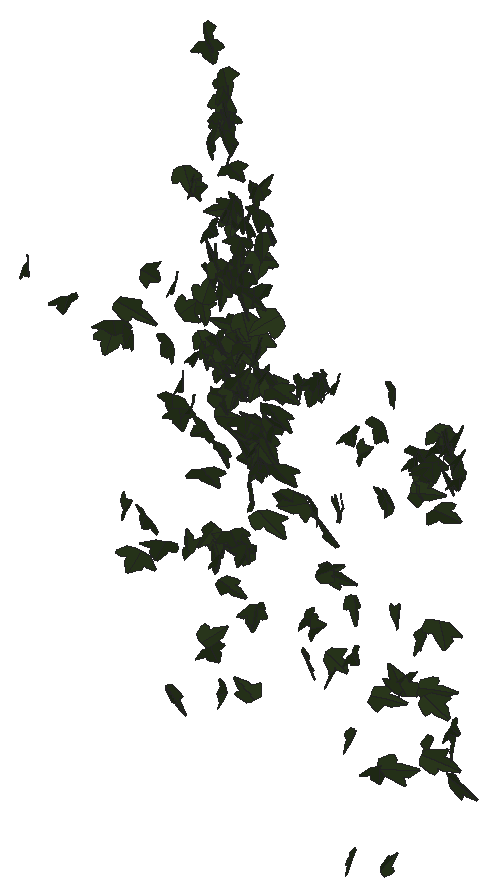
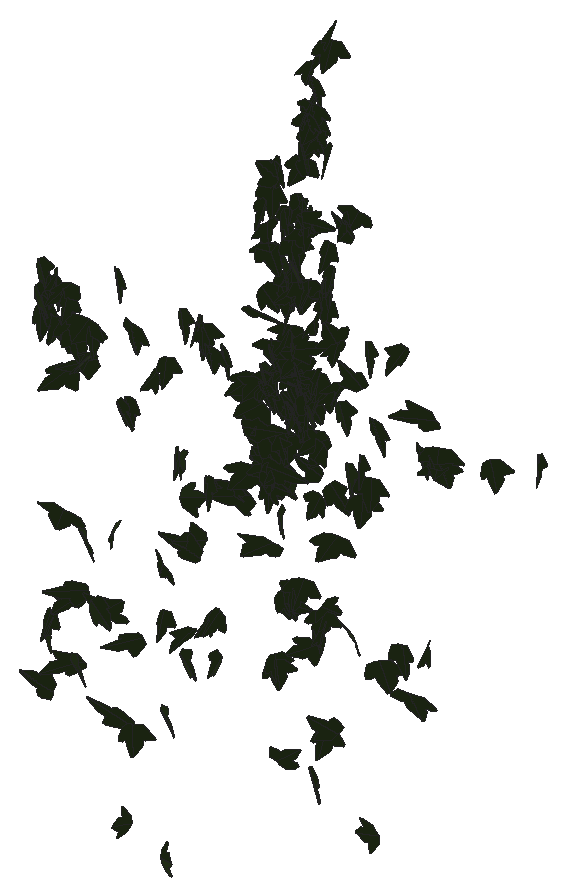
# SketchUp Ruby script. Lengths in millimetres.
U = 1.mm
M = Sketchup.active_model
def pt(a) = Geom::Point3d.new(a.map { |v| v * U })
def face(e, loops, mat)
  f = e.add_face(loops[0].map { |a| pt(a) })
  loops[1..].each { |l| e.add_face(l.map { |a| pt(a) }).erase! }
  f.material = f.back_material = mat if mat
  f
end
# faces: each face lists its corners as indices into pts; further lists are holes
def faces(e, pts, list, mat = nil) = list.each { |f| face(e, (f[0].is_a?(Array) ? f : [f]).map { |l| l.map { |i| pts[i] } }, mat) }
# xy, xz, yz: faces in a plane at the given z, y or x. An outline is a flat list of corners, or four numbers for a rectangle; further outlines are holes
def ring(l) = l.size == 4 ? [[l[0], l[1]], [l[2], l[1]], [l[2], l[3]], [l[0], l[3]]] : l.each_slice(2).to_a
def flat(e, list, mat, &to3) = list.each { |f| face(e, (f[0].is_a?(Array) ? f : [f]).map { |l| ring(l).map { |u, v| to3.(u, v) } }, mat) }
def xy(e, z, list, mat = nil) = flat(e, list, mat) { |x, y| [x, y, z] }
def xz(e, y, list, mat = nil) = flat(e, list, mat) { |x, z| [x, y, z] }
def yz(e, x, list, mat = nil) = flat(e, list, mat) { |y, z| [x, y, z] }
def lines(e, pts, list) = list.each { |a, b| e.add_line(pt(pts[a]), pt(pts[b])) }
# prism: a flat outline (further loops are holes) pulled along v
def prism(e, loops, v, mat = nil)
  f = face(e, loops, mat); d = Geom::Vector3d.new(v.map { |x| x * U })
  f.pushpull(f.normal.samedirection?(d) ? d.length : -d.length)
end
def box(e, o, s, mat = nil) = prism(e, [[o, [o[0] + s[0], o[1], o[2]], [o[0] + s[0], o[1] + s[1], o[2]], [o[0], o[1] + s[1], o[2]]]], [0, 0, s[2]], mat)
def at(x, y, z, deg = 0) = Geom::Transformation.translation(pt([x, y, z])) * Geom::Transformation.rotation(ORIGIN, Z_AXIS, deg.degrees)
def axes(o, x, y, z) = Geom::Transformation.new([*x, 0, *y, 0, *z, 0, *pt(o).to_a, 1])
def part(name) = M.definitions.add(name)
# library, detail: a bought-in or finely detailed component or shape, given as its bounding box
def library(name, o, s) = part(name).tap { |d| box(d.entities, o, s) }
def detail(e, o, s) = box(e.add_group.entities, o, s)
def put(e, d, t, mat = nil) = e.add_instance(d, t).tap { |i| i.material = mat if mat }
def group(e, t, mat = nil) = e.add_group.tap { |g| g.transformation = t; g.material = mat if mat }.entities
root = M.entities
M.materials.add("efeu2").color = [43, 57, 29]
c1 = part("ivyleaf_10")
p = [[0,12.8,-0.8],[-1.5,51.3,-10.9],[-4.9,51,-11.6],[-13.6,26.5,-7.3],[-13.2,15.9,-4.6],[-21.1,19.3,-7.2],
  [-29.5,16.3,-8.3],[-29.2,8.3,-6.2],[-19.7,-9.8,0.5],[-7.6,-13,4],[1,-12.2,5.8],[-0.4,51.1,-11.1],
  [-1.5,51.1,-10.9],[1,-12.4,5.9],[16.9,-12.4,3.5],[35.1,9.1,-5.1],[35,12.9,-6.1],[20.5,16.4,-4.9],
  [15.8,15,-3.8],[15.3,27.6,-7.1],[12.8,31.3,-7.8]]
faces(c1.entities,p,[[0,1,2,3,4,5,6,7,8,9,10],[11,12,0,13,14,15,16,17,18,19,20]],"efeu2")
put(root,c1,axes([392.9,1061.3,793.9],[0.22328,-0.58138,-0.2462],[0.15253,0.26211,-0.58075],[1.1919,0.07537,0.12044]))
put(root,c1,axes([469.6,1064.6,759.5],[-0.40368,-0.59835,-0.04185],[0.01906,0.04086,-0.63482],[1.1414,-0.2123,-0.0042]))
put(root,c1,axes([556.4,1064.1,726.9],[0.80132,0.45198,-0.16049],[-0.25562,-0.09391,-0.61682],[-0.87632,0.44069,0.03316]))
put(root,c1,axes([561.7,1063.9,746.8],[-0.80907,-0.46934,-0.09728],[0.14828,0.06064,-0.63302],[0.90009,-0.43186,0.01684]))
put(root,c1,axes([585,1057,439.4],[0.06877,-0.15139,-0.63183],[0.06726,0.63232,-0.14948],[1.2347,-0.02602,0.04333]))
put(root,c1,axes([589.1,1063.6,739.4],[0.76379,-0.46532,-0.1728],[-0.03848,0.2067,-0.60357],[0.9439,0.38495,0.11522]))
put(root,c1,axes([607.7,1062.6,361.6],[1.193,-0.04431,-0.10252],[-0.19466,0.00702,-0.6284],[0.08538,0.63513,-0.0002]))
put(root,c1,axes([585.9,1058.6,789.2],[0.43486,0.10897,0.60259],[1.0456,0.24761,-0.25309],[-0.51477,0.59499,-0.00503]))
put(root,c1,axes([622.1,1067,428.7],[-0.86457,0.31996,0.33371],[-0.55477,0.16492,-0.55492],[-0.68296,-0.53901,0.02831]))
put(root,c1,axes([635.3,1050.3,868.7],[0.12233,0.43176,0.51307],[-0.17473,0.51623,-0.42292],[-1.2642,-0.02957,0.1081]))
put(root,c1,axes([654,1068.2,393.3],[-0.77826,-0.47441,0.11149],[-0.12473,-0.09068,-0.62625],[0.91906,-0.41403,0.00942]))
put(root,c1,axes([668.9,1061.3,749.4],[0.7785,-0.43948,-0.31281],[-0.20694,0.31734,-0.58803],[1.00559,0.40554,0.12116]))
put(root,c1,axes([678.7,1062.8,658.7],[-0.84104,-0.1225,0.08321],[-0.09056,-0.05701,-0.69887],[0.15634,-0.69204,0.04284]))
put(root,c1,axes([680.3,1062.5,864.1],[0.16723,-0.62621,-0.30183],[-0.09446,0.29198,-0.64093],[0.84282,0.15698,-0.01195]))
put(root,c1,axes([665.8,1073.2,138.9],[-0.44881,0.29664,-0.51951],[0.58109,-0.42054,-0.37872],[-0.97912,-0.38556,0.01337]))
put(root,c1,axes([685.9,1069.2,634.1],[-0.59843,-0.48389,-0.056],[0.06209,0.02813,-0.68884],[0.59103,-0.4929,0.01566]))
put(root,c1,axes([688.2,1068.5,691.8],[0.1738,-0.5851,-0.3012],[0.09152,0.30921,-0.58608],[1.24911,0.05876,0.08485]))
put(root,c1,axes([691.2,1072.2,811.6],[0.62877,-0.01901,-0.45169],[0.54909,-0.04296,0.51536],[-0.05196,-0.68396,-0.01982]))
put(root,c1,axes([715.1,1054.2,410.7],[0.54478,-0.018,0.5821],[-0.58554,0.40411,0.38067],[-0.40244,-0.61232,0.23412]))
put(root,c1,axes([698.8,1062.4,1059.8],[0.72653,0.1688,0.28357],[0.32911,0.08796,-0.61889],[-0.23189,0.65369,0.01006]))
put(root,c1,axes([711.3,1076.8,1048.2],[-0.05253,0.44145,-0.49501],[-0.08526,-0.49631,-0.43653],[-0.80468,0.02377,0.07857]))
put(root,c1,axes([716.4,1058.1,665.1],[0.0959,-0.56776,-0.30934],[-0.05063,0.30819,-0.57],[1.2295,0.05698,0.00066]))
put(root,c1,axes([705.4,1074.6,1034.9],[0.26849,-0.13751,-0.61151],[0.61981,-0.34043,0.25939],[-0.44783,-0.55361,-0.00761]))
put(root,c1,axes([726.4,1061.4,756.1],[-0.03635,-0.63454,-0.11075],[-0.02695,0.11119,-0.63459],[1.22561,-0.01637,-0.01724]))
put(root,c1,axes([741.9,1060.7,627.3],[-0.50209,-0.0235,0.53432],[-0.65103,-0.02726,-0.41222],[0.04385,-0.67389,-0.00195]))
put(root,c1,axes([734.3,1058.4,787.1],[0.20787,0.6266,0.06189],[-0.00518,0.06328,-0.6359],[-1.19833,0.10842,0.01348]))
put(root,c1,axes([736.9,1059.4,845.7],[0.12372,0.63143,0.01278],[-0.002,0.01321,-0.63951],[-0.7705,0.10135,0.00371]))
put(root,c1,axes([747,1063.4,940.4],[-0.5422,0.30795,0.35546],[-0.34994,0.21008,-0.54064],[-0.4547,-0.5289,-0.00778]))
put(root,c1,axes([737.9,1061.6,857.1],[0.39649,0.52898,-0.35342],[0.23779,0.29499,0.62075],[0.73881,-0.37882,-0.01013]))
put(root,c1,axes([738.6,1063,552.5],[-0.88042,-0.35241,-0.27711],[0.41422,0.17158,-0.58153],[0.74594,-0.51122,-0.00415]))
put(root,c1,axes([745.4,1060.9,954.8],[-0.57024,0.42153,0.17021],[-0.14614,0.1213,-0.62934],[-0.53501,-0.48242,-0.00952]))
put(root,c1,axes([742.6,1059.3,771.6],[0.11317,0.63243,-0.06084],[-0.09823,-0.0561,-0.63356],[-1.20521,0.06396,0.04593]))
put(root,c1,axes([743.5,1061.7,1324.2],[-0.24073,0.68446,0.04343],[-0.01136,0.04251,-0.71233],[-0.83664,-0.19752,-0.00282]))
put(root,c1,axes([745.2,1062.9,1297.6],[-0.5946,-0.48443,-0.14762],[0.16886,0.06966,-0.68556],[0.59431,-0.50445,0.04709]))
put(root,c1,axes([749.9,1063.5,905.3],[-0.73336,0.18282,0.11682],[-0.1341,0.04004,-0.62827],[-0.22819,-0.61105,-0.00621]))
put(root,c1,axes([748.7,1069.7,451.7],[0.23452,0.36446,-0.49963],[-0.26019,-0.45204,-0.41181],[-0.7082,0.28677,-0.01415]))
put(root,c1,axes([754.9,1054.3,1131.8],[-0.25245,0.39976,0.54185],[-0.37287,0.44934,-0.44822],[-0.73199,-0.36676,0.04145]))
put(root,c1,axes([750.5,1071.2,437.9],[-0.61943,-0.42061,-0.14316],[0.26525,-0.04563,-0.63706],[0.47272,-0.52555,0.16988]))
put(root,c1,axes([751.1,1072.8,416.5],[-0.10583,0.61072,-0.17549],[0.03365,-0.17333,-0.61684],[-0.77449,-0.09098,-0.00282]))
put(root,c1,axes([755,1054.4,985.6],[-0.08017,-0.50292,-0.45112],[0.07236,0.4472,-0.50719],[0.82105,-0.08852,0.00065]))
put(root,c1,axes([753.7,1078.6,1160],[0.16363,0.55805,-0.35439],[-0.13116,-0.33838,-0.57353],[-0.79576,0.17053,0.02166]))
put(root,c1,axes([762,1061,921.1],[-0.15887,0.29519,-0.60342],[-0.26362,0.56358,0.32233],[0.77598,0.25189,-0.01404]))
put(root,c1,axes([743.1,1061.5,263.6],[0.4158,0.20985,-0.55696],[0.59238,0.27314,0.40004],[0.41993,-0.59309,-0.01284]))
put(root,c1,axes([755.7,1057.9,251.7],[-0.43025,-0.55517,-0.29055],[0.25785,0.25826,-0.5989],[1.16435,-0.26234,0.02526]))
put(root,c1,axes([756,1072,689.7],[-0.71044,0.29558,-0.19809],[0.21399,-0.0921,-0.65304],[-0.3777,-0.60816,0.00262]))
put(root,c1,axes([764.5,1064.6,412.5],[0.08432,-0.65577,-0.06218],[-0.00676,0.06194,-0.6594],[0.8036,0.06933,0.00098]))
put(root,c1,axes([767.5,1062.7,789.6],[-0.80006,-0.02069,0.03525],[-0.04267,-0.00937,-0.65606],[0.02582,-0.65667,0.00825]))
put(root,c1,axes([767.8,1062.1,793.5],[-0.28795,0.50899,0.31432],[-0.19706,0.27113,-0.56034],[-0.70273,-0.28459,0.02834]))
put(root,c1,axes([761,1060.3,694.6],[0.29358,0.15755,0.56905],[0.2357,0.55966,-0.23664],[-0.6807,0.26174,0.16348]))
put(root,c1,axes([766.1,1064.2,605],[-0.69626,0.2669,-0.16946],[0.1823,-0.08047,-0.62996],[-0.33991,-0.58987,0.00926]))
put(root,c1,axes([781.1,1070.3,1023.7],[0.23337,0.08868,-0.65033],[-0.72864,-0.2574,-0.21077],[-0.33207,0.62711,0.00545]))
put(root,c1,axes([766.9,1071,877.1],[0.01214,0.56322,-0.30632],[0.00296,-0.30639,-0.56327],[-0.78218,0.00758,-0.00689]))
put(root,c1,axes([765.5,1071.8,1202.1],[0.83127,-0.00889,0.07959],[0.09713,0.00142,-0.68142],[0.01057,0.686,0.00244]))
put(root,c1,axes([777.8,1058.1,183.7],[0.28392,-0.45395,-0.49396],[-0.28257,0.47114,-0.47781],[1.24514,0.21043,0.0042]))
put(root,c1,axes([771.6,1065.3,747.6],[-0.58516,0.5382,0.14897],[-0.13809,0.13012,-0.61983],[-1.0538,-0.3159,-0.0015]))
put(root,c1,axes([772.6,1070.6,749.3],[-0.17042,0.33649,0.52486],[0.06826,-0.52893,0.354],[0.75755,0.12336,0.08617]))
put(root,c1,axes([773.1,1063.8,1235],[0.71357,-0.38305,-0.11515],[-0.0825,0.10636,-0.69728],[0.48096,0.58655,0.05124]))
put(root,c1,axes([779.7,1064.6,752.9],[-0.48282,-0.51057,0.28851],[-0.197,-0.23974,-0.64575],[0.68781,-0.42707,0.01757]))
put(root,c1,axes([771.7,1068.3,1178.9],[-0.7696,-0.25518,-0.17458],[0.22699,0.00349,-0.67742],[0.30125,-0.65452,0.06445]))
put(root,c1,axes([765.1,1077,732.3],[0.41577,-0.44059,-0.36727],[0.28085,-0.28622,0.55698],[-0.64095,-0.41122,0.00583]))
put(root,c1,axes([774,1069.1,1150.8],[-0.7642,0.27097,-0.10557],[0.08173,-0.10952,-0.67857],[-0.34524,-0.62572,0.07305]))
put(root,c1,axes([771.5,1074.5,1187.8],[0.72901,-0.29129,0.15191],[0.1723,-0.05691,-0.66468],[0.36187,0.61392,0.01046]))
put(root,c1,axes([761.3,1073,652.9],[0.25646,-0.04963,-0.60136],[0.70436,-0.1686,0.21573],[-0.21402,-0.61433,-0.01062]))
put(root,c1,axes([775,1067.2,1202],[-0.29686,0.63919,-0.06217],[0.01456,-0.06197,-0.68385],[-0.78336,-0.24338,0.01085]))
put(root,c1,axes([766.3,1058.7,921.1],[0.63936,0.15019,0.40597],[0.46734,0.13593,-0.54479],[-0.24591,0.64883,0.02016]))
put(root,c1,axes([777.7,1059.6,778.9],[-1.02579,-0.33163,-0.13671],[0.32068,-0.01623,-0.62491],[0.60267,-0.55581,0.09981]))
put(root,c1,axes([779.7,1073.5,1174.7],[-0.23363,0.5091,0.4197],[0.18122,-0.39254,0.54393],[0.78429,0.24236,-0.00065]))
put(root,c1,axes([777.1,1076.8,1109.3],[0.23756,-0.63629,-0.13979],[0.04709,-0.13438,0.66541],[-0.79339,-0.19849,-0.00237]))
put(root,c1,axes([795.1,1066.3,825.7],[-0.11304,-0.03208,-0.65813],[-0.75864,-0.21552,0.09806],[-0.26583,0.62871,0.00003]))
put(root,c1,axes([779.5,1060.3,1259],[0.07041,0.70095,0.01442],[0.00305,0.01426,-0.70332],[-0.85534,0.05775,-0.00132]))
put(root,c1,axes([786.9,1055.7,914.4],[-0.15792,0.28389,0.59825],[-0.32037,0.53759,-0.31192],[-0.74164,-0.29267,0.00736]))
put(root,c1,axes([783.8,1058.1,1013.7],[0.14046,-0.47739,0.43153],[-0.139,0.41633,0.49098],[-0.77269,-0.16167,-0.00988]))
put(root,c1,axes([787.9,1067.4,724.6],[-0.6433,0.41618,0.11689],[-0.16659,0.01458,-0.66787],[-0.50039,-0.5399,0.07207]))
put(root,c1,axes([783.2,1071.4,1007.4],[0.44064,0.5389,-0.07464],[-0.04636,-0.06438,-0.64873],[-0.66211,0.36315,-0.00424]))
put(root,c1,axes([801.9,1055.1,1018.1],[-0.08021,0.01768,0.64973],[-0.76433,0.1722,-0.06808],[-0.21119,-0.62994,-0.00037]))
put(root,c1,axes([793,1060.8,913.8],[-0.7415,-0.23896,0.03297],[-0.03543,-0.01623,-0.65306],[0.29215,-0.60847,0.00447]))
put(root,c1,axes([782.9,1061.9,776.9],[0.77544,0.46805,0.16624],[0.1815,0.1373,-0.6203],[-0.92772,0.41808,0.01759]))
put(root,c1,axes([781.5,1058.6,375.6],[-0.4603,-0.06423,-0.52016],[0.63382,0.03877,-0.38162],[0.0844,-0.64141,0.02902]))
put(root,c1,axes([790.4,1067.7,710.9],[0.82191,0.02357,-0.00614],[-0.00652,-0.02288,-0.67373],[-0.029,0.67334,-0.02268]))
put(root,c1,axes([794.1,1066.3,1037.3],[0.03141,0.53188,-0.34971],[-0.15073,-0.33917,-0.52493],[-0.76182,0.08904,0.08944]))
put(root,c1,axes([802.6,1059.4,1044.1],[-0.6156,0.26111,0.3322],[-0.42688,0.03184,-0.55651],[-0.28897,-0.60329,0.11441]))
put(root,c1,axes([793.2,1059.7,1103.2],[-0.54905,-0.36453,-0.3079],[0.28174,0.20398,-0.57904],[0.50942,-0.5057,-0.01161]))
put(root,c1,axes([795.4,1060.6,464.7],[-0.6033,-0.47064,-0.21459],[0.22205,0.11957,-0.68166],[0.59069,-0.52563,0.03708]))
put(root,c1,axes([800.5,1066,793.6],[0.40324,-0.5172,-0.22841],[-0.13116,0.20225,-0.61355],[0.67719,0.34715,0.01717]))
put(root,c1,axes([806.4,1064.8,971.8],[0.43366,-0.15738,-0.51242],[-0.3594,0.45631,-0.3445],[0.54635,0.42509,0.1801]))
put(root,c1,axes([790,1074.9,937.2],[-0.0351,-0.22617,-0.60564],[0.43311,-0.51218,0.17441],[-0.65917,-0.32449,0.14684]))
put(root,c1,axes([816.7,1069.4,436.1],[0.04863,0.04852,-0.64974],[-0.79459,0.02068,-0.03841],[0.02163,0.65063,0.04968]))
put(root,c1,axes([807.4,1063.2,977.8],[-0.58937,-0.39821,0.12112],[-0.11654,-0.07454,-0.62605],[0.49424,-0.49243,-0.00318]))
put(root,c1,axes([810.7,1055,821.9],[0.19771,-0.13127,0.63158],[-0.61394,0.54341,0.166],[-1.06318,-0.33821,0.02159]))
put(root,c1,axes([795.1,1057.1,804.7],[0.44567,0.40188,0.4552],[0.1708,0.45962,-0.45195],[-1.14298,0.22539,0.10996]))
put(root,c1,axes([802.3,1067.1,722.9],[0.53399,-0.51157,0.11609],[0.07989,-0.09673,-0.67314],[0.63497,0.44238,-0.01294]))
put(root,c1,axes([804.8,1073.3,711.3],[-0.45505,0.49609,0.18125],[0.1256,-0.14935,0.62062],[0.632,0.38687,0.00717]))
put(root,c1,axes([806.9,1064.1,782.1],[0.35691,-0.60033,-0.10885],[-0.01037,0.11222,-0.62832],[1.16113,0.18553,0.02785]))
put(root,c1,axes([807.2,1060.8,774.1],[-0.47531,-0.51808,-0.01696],[0.0236,0.00667,-0.64812],[0.63195,-0.38991,0.01145]))
put(root,c1,axes([801.8,1057.1,726.9],[-0.23832,-0.54751,0.36877],[0.1355,0.35184,0.5812],[-0.79387,0.22441,-0.01151]))
put(root,c1,axes([815.7,1059.5,924],[-0.77753,-0.16943,0.08223],[-0.09629,-0.02317,-0.65945],[0.20861,-0.64219,0.0021]))
put(root,c1,axes([816.5,1067.7,444.4],[-0.2957,-0.60548,0.22694],[-0.09696,-0.21263,-0.65217],[0.78289,-0.25502,0.00495]))
put(root,c1,axes([808.8,1059.4,903.1],[-0.0483,-0.08426,-0.63753],[0.26965,0.59804,-0.09277],[0.73675,-0.2244,-0.00785]))
put(root,c1,axes([808.2,1069.4,455.3],[-0.58935,0.34353,-0.33091],[0.24146,-0.28416,-0.58391],[-0.52946,-0.51197,0.10205]))
put(root,c1,axes([808.1,1064.2,625.8],[-0.65058,0.50423,-0.18434],[0.19542,-0.15309,-0.60918],[-1.00292,-0.35692,0.00088]))
put(root,c1,axes([814.3,1054,929.5],[0.0981,-0.04179,-0.68303],[0.03738,0.68726,-0.03844],[0.83402,-0.02589,0.08207]))
put(root,c1,axes([837,1069.8,631.8],[-0.0146,0.03151,-0.64129],[-1.15093,0.21513,0.0178],[0.41058,0.60417,0.0271]))
put(root,c1,axes([816.2,1066.3,1019],[0.04919,-0.63697,-0.09723],[-0.0145,0.09667,-0.63822],[0.78597,0.04165,-0.00569]))
put(root,c1,axes([817.4,1070.8,947.5],[0.2895,-0.54857,-0.22597],[-0.11525,0.20534,-0.59767],[0.71458,0.25536,-0.00484]))
put(root,c1,axes([817.8,1067.5,729.4],[0.44203,-0.51699,-0.24102],[-0.10004,0.23535,-0.62812],[0.68868,0.36603,0.06345]))
put(root,c1,axes([818.1,1058.2,873],[-0.43803,0.52398,0.21858],[-0.15087,0.18023,-0.63519],[-0.67601,-0.37974,0.00013]))
put(root,c1,axes([819.1,1066.8,817.9],[0.0845,0.64521,-0.07355],[-0.0299,0.07651,0.64811],[0.79169,-0.06597,0.03233]))
put(root,c1,axes([825.7,1065.6,193.3],[0.49524,0.26107,0.41751],[-0.46386,-0.17765,0.48076],[0.38174,-0.55456,0.04254]))
put(root,c1,axes([820.4,1059.1,674.5],[-0.49563,-0.55467,-0.06132],[0.05174,0.04495,-0.68749],[0.67885,-0.40839,0.00762]))
put(root,c1,axes([822.6,1058.9,1017],[-0.66939,0.35966,0.15997],[-0.16621,0.08396,-0.65604],[-0.45055,-0.56532,0.00434]))
put(root,c1,axes([814.4,1061.3,845.5],[0.58601,0.4413,0.14869],[0.12333,0.1097,-0.65217],[-0.55458,0.49071,0.01208]))
put(root,c1,axes([811.5,1061.2,790.4],[0.40576,0.39263,0.41411],[0.31732,0.32233,-0.51451],[-0.61967,0.42215,0.00769]))
put(root,c1,axes([815.6,1058.3,805.6],[-0.37162,-0.42206,-0.45564],[0.55891,0.35812,-0.45757],[1.04155,-0.34276,0.08297]))
put(root,c1,axes([839.5,1057.7,610.7],[-0.29227,0.05717,0.6395],[-0.78307,-0.00475,-0.24002],[-0.01903,-0.68288,0.05521]))
put(root,c1,axes([829,1070.9,335.1],[-0.49247,-0.50379,0.07924],[0.04194,-0.12771,-0.63682],[0.62076,-0.39104,0.10589]))
put(root,c1,axes([837.7,1072.1,668.6],[-0.58755,-0.29861,0.35694],[-0.30636,-0.26572,-0.56111],[0.47801,-0.53734,0.07912]))
put(root,c1,axes([831,1070,343.9],[-0.25237,-0.62156,0.06595],[0.09237,-0.09387,-0.64725],[0.75695,-0.19578,0.10097]))
put(root,c1,axes([841,1047,546.3],[-0.00541,-0.01683,-0.71011],[-0.25082,0.6978,-0.01601],[1.32839,0.13168,-0.00592]))
put(root,c1,axes([851.3,1062.1,600.3],[-0.23842,0.16685,-0.62025],[-0.80305,0.45507,0.20764],[0.92164,0.43968,0.02047]))
put(root,c1,axes([817.8,1063.2,887.1],[0.26225,-0.05663,0.60563],[0.72582,0.15335,-0.19683],[-0.15455,0.62408,0.10332]))
put(root,c1,axes([832.4,1069.4,740.6],[0.80707,-0.13423,-0.04557],[-0.05376,0.01198,-0.67501],[0.16437,0.66299,0.00297]))
put(root,c1,axes([836.8,1054.8,615.9],[0.11995,-0.05618,0.67062],[-0.3152,0.65154,0.07015],[-1.2414,-0.17086,0.04699]))
put(root,c1,axes([844,1068.8,958.9],[-0.70886,-0.23408,0.27559],[-0.30209,-0.12253,-0.62612],[0.32147,-0.6313,0.01933]))
put(root,c1,axes([835.8,1062.3,1079.7],[-0.68518,0.32027,-0.13788],[0.03915,-0.21283,-0.62504],[-0.4236,-0.53771,0.16527]))
put(root,c1,axes([841.4,1078.2,899.9],[-0.11682,-0.59082,0.30295],[-0.05314,-0.29983,-0.59851],[0.80828,-0.1051,0.00444]))
put(root,c1,axes([840.2,1062.9,797.8],[0.50863,-0.58261,-0.0424],[-0.01779,0.04235,-0.64092],[1.11162,0.26726,0.00914]))
put(root,c1,axes([839,1069.2,809.7],[0.3619,-0.61041,0.08633],[0.08229,-0.06309,-0.67787],[0.74759,0.30243,0.03283]))
put(root,c1,axes([837.1,1069.2,818.2],[0.76103,0.28945,0.00194],[0.00846,-0.01033,-0.68757],[-0.35304,0.62371,-0.01229]))
put(root,c1,axes([842.6,1064.3,607.3],[0.16495,0.61816,-0.31897],[-0.25824,-0.27297,-0.61873],[-0.80839,0.21333,0.13257]))
put(root,c1,axes([839.6,1064.4,1069.8],[-0.00145,-0.56757,0.4258],[0.00084,0.4258,0.56757],[-0.86563,0.00136,-0.00016]))
put(root,c1,axes([848,1058.8,1042.8],[-0.85795,0.07976,0.12362],[-0.1582,-0.05094,-0.70482],[-0.08477,-0.7122,0.06426]))
put(root,c1,axes([845.7,1066.7,600.8],[-0.07536,-0.69089,-0.10099],[0.09031,0.09433,-0.69063],[0.84705,-0.07153,0.06465]))
put(root,c1,axes([843,1066.7,960.5],[0.71999,0.3555,-0.04267],[-0.04825,-0.01704,-0.68894],[-0.43415,0.59145,0.0058]))
put(root,c1,axes([846.2,1073.3,623.7],[-0.04235,-0.32985,0.54581],[0.12843,-0.54208,-0.3209],[0.76736,0.07253,0.08383]))
put(root,c1,axes([849.2,1071.4,749.6],[0.75635,-0.2508,-0.17565],[-0.18562,0.09191,-0.66822],[0.32418,0.63778,0.02722]))
put(root,c1,axes([834.4,1063.8,631],[-0.91551,0.0488,-0.42972],[0.81249,-0.0493,-0.48348],[-0.13174,-0.64314,0.00446]))
put(root,c1,axes([847.8,1067.5,993.5],[0.10474,0.68528,-0.11861],[-0.10756,-0.10782,-0.68676],[-0.84162,0.09907,0.07301]))
put(root,c1,axes([847.6,1066.7,759.6],[-0.74069,0.26115,-0.10228],[0.11567,-0.03841,-0.6609],[-0.32202,-0.61448,-0.00215]))
put(root,c1,axes([873.8,1063.8,677.2],[-0.31335,0.16467,-0.61021],[-1.20051,-0.00309,0.16936],[0.07577,0.63203,0.15982]))
put(root,c1,axes([847.7,1066.7,758.3],[-0.7527,0.11882,-0.22736],[0.26208,-0.08443,-0.62704],[-0.17108,-0.65208,0.03976]))
put(root,c1,axes([867,1070.3,858.6],[-0.83527,0.30675,0.33162],[-0.52029,-0.63747,-0.29081],[0.18174,-0.41515,0.69157]))
put(root,c1,axes([858.1,1060.7,767.4],[0.20607,-0.62752,-0.10166],[-0.0434,0.09922,-0.63677],[1.20908,0.11051,-0.00553]))
put(root,c1,axes([855.8,1068.6,1020.7],[-0.59661,0.49137,0.06251],[-0.04627,0.05045,-0.69319],[-0.60253,-0.49041,-0.00867]))
put(root,c1,axes([847.2,1060.6,634.9],[0.60127,0.10314,0.51001],[0.59443,0.15507,-0.5022],[-0.2228,0.69207,0.03652]))
put(root,c1,axes([849.1,1067,510.5],[0.79716,0.30393,0.38857],[0.57704,0.24349,-0.51728],[-0.74061,0.51685,0.0152]))
put(root,c1,axes([857.7,1063.3,653.4],[-0.6812,0.16877,-0.41205],[0.41351,-0.2675,-0.56886],[-0.35229,-0.64031,0.12904]))
put(root,c1,axes([862,1067.1,747.9],[0.54735,0.33923,0.36591],[0.35456,0.22233,-0.56245],[-0.49482,0.53455,0.00173]))
put(root,c1,axes([873,1046.3,679.5],[0.21373,-0.02585,-0.67985],[0.10492,0.68713,-0.01702],[1.29056,-0.05158,0.11398]))
put(root,c1,axes([872.7,1059.9,709.4],[-1.02922,0.16487,-0.30269],[0.53762,-0.11071,-0.56498],[-0.3759,-0.60976,0.02074]))
put(root,c1,axes([879,1062.2,607.6],[-1.02288,-0.21297,-0.30948],[0.53669,0.12822,-0.57795],[0.47241,-0.60679,-0.0135]))
put(root,c1,axes([880.7,1060.7,745.5],[-0.60579,-0.35708,-0.43601],[0.67718,0.261,-0.4735],[0.83179,-0.47255,0.06795]))
put(root,c1,axes([929,1058.2,566],[0.8326,-0.23475,-0.45474],[-0.76994,0.20776,-0.49644],[0.59651,0.59582,-0.00606]))
put(root,c1,axes([897.4,1062.1,566.2],[-0.73638,0.0765,-0.53333],[1.00042,-0.09049,-0.39433],[-0.22501,-0.65265,-0.00784]))
put(root,c1,axes([925,1060.7,771.6],[0.56889,-0.53353,-0.20138],[-0.00251,0.22672,-0.60262],[1.08533,0.28018,0.10416]))
put(root,c1,axes([936.9,1060.4,368],[-0.15788,-0.35065,-0.52599],[0.28982,0.50379,-0.35987],[1.16768,-0.17245,0.0182]))
put(root,c1,axes([938.3,1059.8,301.5],[-0.54659,0.56478,-0.06141],[0.0509,-0.05529,-0.63361],[-1.08002,-0.28844,0.00121]))
put(root,c1,axes([943.9,1064.7,770],[0.98712,-0.36951,0.01274],[0.13427,0.07736,-0.62829],[0.69074,0.51302,0.10392]))
put(root,c1,axes([953,1060.7,563.6],[0.574,-0.36783,-0.45874],[-0.10841,0.49486,-0.43425],[1.11382,0.23773,0.19414]))
put(root,c1,axes([950.4,1059.9,357.9],[0.04874,-0.2422,-0.61075],[0.26539,0.5993,-0.23181],[1.22196,-0.1205,0.07471]))
put(root,c1,axes([958.3,1060.3,793.5],[-0.31601,-0.61112,-0.13191],[0.08695,0.12426,-0.63318],[1.18669,-0.17185,0.01127]))
put(root,c1,axes([966.4,1060.7,787.9],[0.64551,-0.46322,-0.29349],[-0.05613,0.32918,-0.55364],[1.04215,0.30465,0.15197]))
put(root,c1,axes([972.8,1054.6,798.5],[0.27467,-0.5281,-0.3445],[0.2275,0.36991,-0.51698],[1.17826,0.05168,0.18013]))
put(root,c1,axes([992.2,1055.7,525.8],[-0.45416,0.37215,-0.48251],[-0.65311,0.34613,0.43668],[0.95834,0.41225,0.06894]))
put(root,c1,axes([978.4,1049.8,463.6],[0.06296,-0.17729,0.62435],[0.03324,0.62518,0.1766],[-1.23479,0.00779,0.03659]))
put(root,c1,axes([983.5,1070.6,290.9],[0.39642,-0.57579,0.19315],[0.09383,-0.18749,-0.61208],[1.15204,0.2134,-0.01661]))
put(root,c1,axes([996.1,1059.4,800.3],[0.08495,-0.60653,-0.22663],[0.00302,0.22727,-0.60793],[1.23229,0.04126,0.01711]))
put(root,c1,axes([1003.9,1054.3,578],[0.04707,0.12931,-0.63154],[-0.29765,0.61433,0.11967],[1.19024,0.14851,0.0549]))
put(root,c1,axes([973.6,1067.3,455.3],[-0.26212,-0.01356,0.62307],[1.18515,0.02253,0.13814],[-0.04744,0.63771,0.00837]))
put(root,c1,axes([991.2,1054.9,322.5],[0.08213,0.54456,0.35881],[0.07168,0.35691,-0.54621],[-1.23909,0.05674,-0.00781]))
put(root,c1,axes([1006.2,1059.1,587.7],[0.18852,-0.39957,-0.50565],[-0.04205,0.50918,-0.40669],[1.22583,0.07892,0.06381]))
put(root,c1,axes([1020.6,1066.4,191.7],[0.54273,-0.56001,0.1104],[0.08844,-0.10023,-0.62843],[1.08273,0.2889,-0.00401]))
put(root,c1,axes([1023,1060.6,720.6],[-0.22513,-0.58008,-0.2439],[0.16148,0.2312,-0.59104],[1.1867,-0.14151,0.03416]))
put(root,c1,axes([1016.3,1073.3,-20.7],[0.33971,-0.34652,0.51419],[0.43864,-0.45965,-0.38978],[1.09554,0.29149,-0.00338]))
put(root,c1,axes([1026.4,1061,336.8],[-0.06235,-0.53837,-0.3507],[0.19966,0.34196,-0.53476],[1.20643,-0.08442,0.07038]))
put(root,c1,axes([1017.3,1073.1,420.8],[0.73067,-0.33991,0.40081],[0.60949,-0.24226,-0.51219],[0.79305,0.49935,0.02435]))
put(root,c1,axes([1043.2,1058.5,693.6],[0.0242,-0.13437,-0.62764],[0.23404,0.61664,-0.12952],[1.19896,-0.11766,0.03795]))
put(root,c1,axes([1073.2,1068.3,150.5],[-0.50672,-0.58741,-0.11458],[0.09654,0.10281,-0.64493],[1.13494,-0.27101,0.0037]))
put(root,c1,axes([1079.6,1059.4,752.3],[0.94259,-0.41563,-0.07974],[0.05452,0.15539,-0.63201],[0.80361,0.47697,0.13641]))
put(root,c1,axes([1090,1055.3,633.5],[0.67671,-0.39335,-0.35156],[-0.11326,0.39135,-0.49805],[0.99765,0.31124,0.18192]))
put(root,c1,axes([1100.2,1058.5,624.4],[0.13548,-0.16693,-0.61273],[-0.52829,0.54637,-0.1811],[1.08708,0.28632,-0.01165]))
put(root,c1,axes([1077.5,1059.1,281.8],[-0.12379,-0.25527,-0.60484],[0.89536,0.4058,-0.22186],[0.87146,-0.45319,0.14203]))
put(root,c1,axes([1098.1,1052.1,-5.8],[0.09634,-0.23009,0.59352],[-0.30242,0.57197,0.23529],[-1.17314,-0.16634,-0.01191]))
put(root,c1,axes([1106.7,1058.3,823.4],[0.61084,-0.51181,-0.2376],[0.00322,0.27421,-0.5884],[1.07391,0.29029,0.13691]))
put(root,c1,axes([1116.5,1053.1,432.2],[0.12799,0.10616,-0.63271],[-0.05626,0.63602,0.10358],[1.21972,0.01819,0.07117]))
put(root,c1,axes([1092.6,1066.4,158.6],[0.55515,-0.13408,-0.57663],[1.08775,-0.10381,0.31326],[-0.29375,-0.63781,0.07023]))
put(root,c1,axes([1126,1060.9,310.7],[1.13237,0.02493,0.31027],[-0.59001,-0.01268,0.5955],[0.05323,-0.6709,0.00028]))
put(root,c1,axes([1125.5,1079.6,324.1],[0.01601,-0.63597,0.24737],[0.01835,-0.24725,-0.636],[1.29858,0.01134,0.00594]))
put(root,c1,axes([1149.2,1057.8,721.3],[-0.05173,-0.6227,-0.19016],[0.09986,0.18761,-0.62186],[1.23513,-0.04125,0.04231]))
put(root,c1,axes([1160.7,1062.9,412.7],[0.62123,-0.58292,0.02596],[0.02968,-0.02102,-0.66808],[1.11011,0.32677,0.00334]))
put(root,c1,axes([1157.7,1057.7,679.2],[0.37951,-0.21733,-0.57255],[0.33569,0.597,-0.16518],[1.11614,-0.10566,0.24436]))
put(root,c1,axes([1161.3,1062.3,733.1],[-1.19267,0.07208,-0.12786],[0.24392,-0.00456,-0.63072],[-0.13616,-0.63956,-0.00991]))
put(root,c1,axes([1162,1078.2,223.4],[0.60016,-0.56584,0.18487],[0.14693,-0.16857,-0.64763],[1.12336,0.32435,-0.01406]))
put(root,c1,axes([1176.2,1063,709.2],[-0.50392,-0.57937,-0.00286],[-0.00523,0.0044,-0.63699],[1.10266,-0.26475,-0.00433]))
put(root,c1,axes([1160,1050.3,670.5],[-0.07861,-0.18001,-0.6576],[0.8536,0.48901,-0.16203],[0.97728,-0.4416,0.08863]))
put(root,c1,axes([1181.7,1061.5,718.4],[-0.72398,-0.51311,-0.08072],[0.14577,0.04355,-0.63776],[0.97775,-0.38643,0.03531]))
put(root,c1,axes([1168.3,1062.6,326.8],[-0.07139,-0.12566,-0.6279],[0.96516,0.37821,-0.10598],[0.74413,-0.50261,0.07723]))
put(root,c1,axes([1190,1059.4,758.2],[-0.14891,-0.49117,-0.42011],[0.12734,0.41475,-0.49736],[1.22348,-0.10295,0.00063]))
put(root,c1,axes([1179.9,1057.9,309.8],[0.42384,0.48137,0.36426],[0.29424,0.32983,-0.53038],[-1.11056,0.2711,-0.00151]))
put(root,c1,axes([1181.4,1057.4,210.7],[0.27149,0.31111,0.6065],[0.50185,0.54621,-0.34221],[-1.1963,0.29974,-0.00591]))
put(root,c1,axes([1187.2,1065.4,778.2],[-0.32714,-0.49294,-0.36364],[0.63479,0.24147,-0.48499],[0.97783,-0.32167,0.19319]))
put(root,c1,axes([1190.3,1068.4,439],[1.17887,0.02777,0.17996],[0.34083,0.0226,-0.61988],[-0.06273,0.64463,0.01398]))
put(root,c1,axes([1195.5,1059.1,645.6],[-0.46613,-0.38922,-0.54398],[0.66831,0.41823,-0.45734],[1.08348,-0.42542,0.04807]))
put(root,c1,axes([1211.6,1054.4,773.1],[0.45834,-0.49273,-0.37457],[-0.03753,0.39561,-0.53309],[1.17737,0.20443,0.12882]))
put(root,c1,axes([1210.3,1058.2,713.9],[-0.75282,0.50227,0.0222],[-0.02287,0.01879,-0.63932],[-0.95658,-0.39573,-0.00218]))
put(root,c1,axes([1216,1064.4,272.4],[-0.04229,-0.47314,-0.47227],[0.1803,0.46553,-0.47084],[1.25945,-0.08253,0.05155]))
put(root,c1,axes([1213.1,1061.3,783.5],[-0.15591,0.61733,-0.17364],[0.00835,-0.17451,-0.62249],[-1.22047,-0.08005,0.01792]))
put(root,c1,axes([1220.6,1057.1,772],[-0.01693,-0.60241,-0.23675],[0.1154,0.23495,-0.60012],[1.22645,-0.03042,0.0532]))
put(root,c1,axes([1211.5,1074.3,247.3],[0.17672,-0.30136,0.60915],[0.64139,-0.51348,-0.3054],[1.12323,0.34062,0.07855]))
put(root,c1,axes([1233.4,1061.1,794],[0.09978,-0.63569,-0.06027],[0.02274,0.06144,-0.63763],[1.21506,0.05105,0.01688]))
put(root,c1,axes([1235.9,1061.8,754.5],[0.1139,-0.64034,0.01624],[0.00214,-0.01621,-0.64313],[1.21909,0.05985,-0.00039]))
put(root,c1,axes([1232.6,1058.8,742.1],[0.88689,-0.43154,-0.11851],[0.01193,0.17737,-0.62123],[0.85163,0.44692,0.13212]))
put(root,c1,axes([1211.1,1076.3,171.2],[-0.10841,-0.11281,0.64975],[1.21348,-0.176,0.02534],[0.32058,0.62805,0.1238]))
put(root,c1,axes([1237.8,1056.7,719],[-0.17224,-0.59805,-0.24266],[0.04954,0.24145,-0.60478],[1.22733,-0.09367,-0.00964]))
